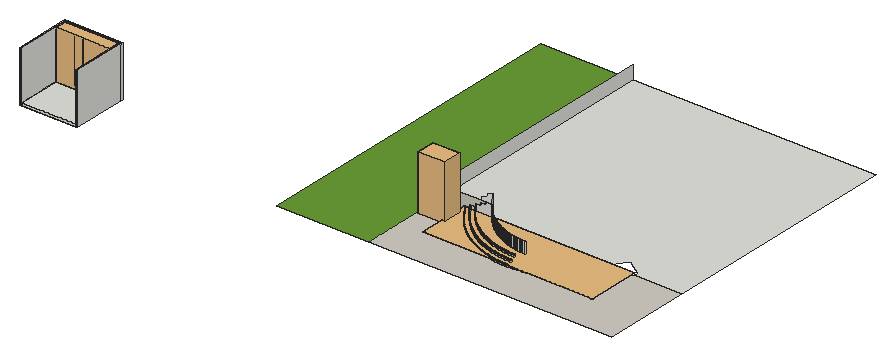
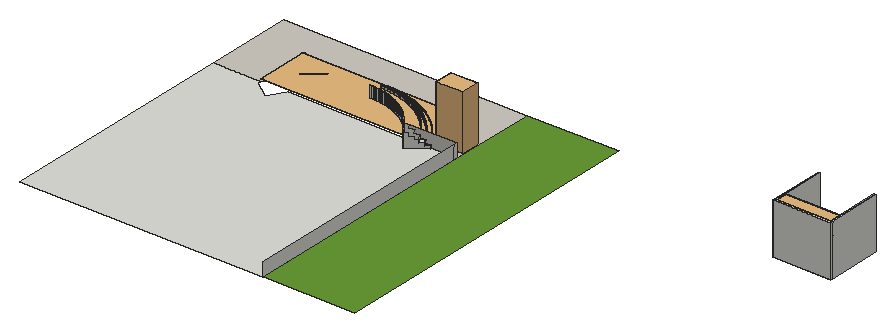
# SketchUp Ruby script. Lengths in inches.
U = 1.inch
M = Sketchup.active_model
def pt(a) = Geom::Point3d.new(a.map { |v| v * U })
def face(e, loops, mat)
  f = e.add_face(loops[0].map { |a| pt(a) })
  loops[1..].each { |l| e.add_face(l.map { |a| pt(a) }).erase! }
  f.material = f.back_material = mat if mat
  f
end
# faces: each face lists its corners as indices into pts; further lists are holes
def faces(e, pts, list, mat = nil) = list.each { |f| face(e, (f[0].is_a?(Array) ? f : [f]).map { |l| l.map { |i| pts[i] } }, mat) }
# xy, xz, yz: faces in a plane at the given z, y or x. An outline is a flat list of corners, or four numbers for a rectangle; further outlines are holes
def ring(l) = l.size == 4 ? [[l[0], l[1]], [l[2], l[1]], [l[2], l[3]], [l[0], l[3]]] : l.each_slice(2).to_a
def flat(e, list, mat, &to3) = list.each { |f| face(e, (f[0].is_a?(Array) ? f : [f]).map { |l| ring(l).map { |u, v| to3.(u, v) } }, mat) }
def xy(e, z, list, mat = nil) = flat(e, list, mat) { |x, y| [x, y, z] }
def xz(e, y, list, mat = nil) = flat(e, list, mat) { |x, z| [x, y, z] }
def yz(e, x, list, mat = nil) = flat(e, list, mat) { |y, z| [x, y, z] }
def lines(e, pts, list) = list.each { |a, b| e.add_line(pt(pts[a]), pt(pts[b])) }
# prism: a flat outline (further loops are holes) pulled along v
def prism(e, loops, v, mat = nil)
  f = face(e, loops, mat); d = Geom::Vector3d.new(v.map { |x| x * U })
  f.pushpull(f.normal.samedirection?(d) ? d.length : -d.length)
end
def box(e, o, s, mat = nil) = prism(e, [[o, [o[0] + s[0], o[1], o[2]], [o[0] + s[0], o[1] + s[1], o[2]], [o[0], o[1] + s[1], o[2]]]], [0, 0, s[2]], mat)
def at(x, y, z, deg = 0) = Geom::Transformation.translation(pt([x, y, z])) * Geom::Transformation.rotation(ORIGIN, Z_AXIS, deg.degrees)
def axes(o, x, y, z) = Geom::Transformation.new([*x, 0, *y, 0, *z, 0, *pt(o).to_a, 1])
def part(name) = M.definitions.add(name)
# library, detail: a bought-in or finely detailed component or shape, given as its bounding box
def library(name, o, s) = part(name).tap { |d| box(d.entities, o, s) }
def detail(e, o, s) = box(e.add_group.entities, o, s)
def put(e, d, t, mat = nil) = e.add_instance(d, t).tap { |i| i.material = mat if mat }
def group(e, t, mat = nil) = e.add_group.tap { |g| g.transformation = t; g.material = mat if mat }.entities
root = M.entities
M.materials.add("Arta-Ceramic-Moonstone-White-24x24-4K").color = [209, 205, 196]
M.materials.add("[Color M09]1").color = [0, 0, 0]
M.materials.add("[Grass Dark Green]").color = [106, 157, 55]
M.materials.add("[Groundcover Gravel 1 inch]").color = [152, 133, 110]
M.materials.add("[Translucent Glass Gray]1").color = [128, 128, 128]
M.materials["[Translucent Glass Gray]1"].alpha = 0.5
c1 = library("Group\#160",[0,-1,0],[120,25,108])
c2 = library("Senza",[-37.85,-41.61,-2.42],[41.39,41.83,53.67])
c3 = library("Mesh Light\#9",[-0.5,-0.5,-0.1],[1,1,0.2])
xy(root,0,[[777.4375,194.875,777.4375,734.875,1318.21,734.875,1318.21,733.875,1318.125,733.875,1318.125,194.875,1212.72,194.875,1216.84,200.64,1177.16,229.03,1152.72,194.875,895.84,194.875,873.77,225.73,834.08,197.34,835.84,194.875],[835.84,194.875,834.08,197.34,873.77,225.73,895.84,194.875]])
xy(root,0,[[[777.4375,0,777.4375,194.875,835.84,194.875,858.18,163.65,860.54,160.49,862.96,157.37,865.43,154.3,867.97,151.27,870.5625,148.3,873.21,145.375,875.92,142.5,878.68,139.68,881.49,136.92,884.36,134.2,887.27,131.55,890.24,128.95,893.26,126.4,896.32,123.92,899.44,121.49,902.59,119.13,905.8,116.82,909.04,114.58,912.33,112.4,915.66,110.29,919.03,108.24,922.44,106.25,925.89,104.33,929.37,102.47,932.89,100.6875,936.44,98.97,940.03,97.32,943.64,95.73,947.29,94.22,950.96,92.78,954.66,91.41,958.38,90.11,962.13,88.88,965.91,87.72,969.7,86.64,973.51,85.63,977.35,84.69,981.2,83.83,985.0625,83.04,988.94,82.32,992.84,81.68,996.74,81.12,1000.66,80.625,1004.58,80.21,1008.51,79.87,1012.45,79.6,1016.39,79.42,1020.34,79.3,1024.28,79.26,1028.23,79.3,1032.17,79.42,1036.11,79.6,1040.05,79.87,1043.98,80.21,1047.9,80.625,1051.82,81.12,1055.72,81.68,1059.62,82.32,1063.5,83.04,1067.36,83.83,1071.21,84.69,1075.05,85.63,1078.86,86.64,1082.66,87.72,1086.43,88.88,1090.18,90.11,1093.9,91.41,1097.6,92.78,1101.28,94.22,1104.92,95.73,1108.54,97.32,1112.12,98.97,1115.67,100.6875,1119.1875,102.47,1122.67,104.33,1126.12,106.25,1129.53,108.24,1132.9,110.29,1136.23,112.4,1139.52,114.58,1142.76,116.82,1145.97,119.13,1149.125,121.49,1152.24,123.92,1155.3,126.4,1158.32,128.95,1161.29,131.55,1164.21,134.2,1167.07,136.92,1169.89,139.68,1172.65,142.5,1175.35,145.375,1178,148.3,1180.59,151.27,1183.13,154.3,1185.6,157.37,1188.02,160.49,1190.38,163.65,1212.72,194.875,1318.125,194.875,1318.125,0],[811.58,149.53,813.26,149.58,814.86,150.07,816.29,150.95,817.44,152.18,818.23,153.66,818.62,155.3,818.5625,156.98,818.08,158.58,817.19,160.01,815.96,161.16,814.48,161.96,812.85,162.34,811.17,162.28,809.56,161.8,808.13,160.91,806.98,159.6875,806.1875,158.2,805.81,156.57,805.86,154.89,806.35,153.28,807.23,151.85,808.46,150.7,809.9375,149.91]]],"Arta-Ceramic-Moonstone-White-24x24-4K")
xy(root,0,[[573.3125,0,777.4375,732.375]],"[Grass Dark Green]")
xy(root,0,[[811.58,149.53,809.9375,149.91,808.46,150.7,807.23,151.85,806.35,153.28,805.86,154.89,805.81,156.57,806.1875,158.2,806.98,159.6875,808.13,160.91,809.56,161.8,811.17,162.28,812.85,162.34,814.48,161.96,815.96,161.16,817.19,160.01,818.08,158.58,818.5625,156.98,818.62,155.3,818.23,153.66,817.44,152.18,816.29,150.95,814.86,150.07,813.26,149.58]],"[Groundcover Gravel 1 inch]")
xy(root,5,[[834.84,194.875,835.5,195.35,835.84,194.875]],"Arta-Ceramic-Moonstone-White-24x24-4K")
xy(root,6,[[835.84,194.875,847.84,194.875,842.02,203.02,834.08,197.34,835.5,195.35]])
xy(root,6,[[834.84,194.875,835.84,194.875,835.5,195.35]],"Arta-Ceramic-Moonstone-White-24x24-4K")
xy(root,11,[[846.84,194.875,847.5,195.35,847.84,194.875]],"Arta-Ceramic-Moonstone-White-24x24-4K")
xy(root,12,[[847.84,194.875,859.84,194.875,849.96,208.69,842.02,203.02,847.5,195.35]])
xy(root,12,[[846.84,194.875,847.84,194.875,847.5,195.35]],"Arta-Ceramic-Moonstone-White-24x24-4K")
xy(root,17,[[858.84,194.875,859.5,195.35,859.84,194.875]],"Arta-Ceramic-Moonstone-White-24x24-4K")
xz(root,194.875,[[835.84,0,895.84,0,895.84,30,882.84,30,882.84,29,883.84,29,883.84,24,870.84,24,870.84,23,871.84,23,871.84,18,858.84,18,858.84,17,859.84,17,859.84,12,846.84,12,846.84,11,847.84,11,847.84,6,834.84,6,834.84,5,835.84,5]])
xz(root,194.875,[[777.4375,0,835.84,0,835.84,5,834.84,5,834.84,6,847.84,6,847.84,11,846.84,11,846.84,12,859.84,12,859.84,17,858.84,17,858.84,18,871.84,18,871.84,23,870.84,23,870.84,24,883.84,24,883.84,29,882.84,29,882.84,30,777.4375,30]],"Arta-Ceramic-Moonstone-White-24x24-4K")
yz(root,777.4375,[[194.875,0,202.125,30],[202.125,0,734.875,30]])
p = [[1016.39,79.42,5],[1016.39,79.42,0],[1020.34,79.3,0],[1020.34,79.3,5],[1024.28,79.26,0],[1024.28,79.26,5],
  [1012.45,79.6,5],[1012.45,79.6,0],[1008.51,79.87,5],[1008.51,79.87,0],[1004.58,80.21,5],[1004.58,80.21,0],
  [1000.66,80.625,5],[1000.66,80.625,0],[996.74,81.12,5],[996.74,81.12,0],[992.84,81.68,5],[992.84,81.68,0],
  [988.94,82.32,5],[988.94,82.32,0],[985.0625,83.04,5],[985.0625,83.04,0],[981.2,83.83,5],[981.2,83.83,0],
  [977.35,84.69,5],[977.35,84.69,0],[973.51,85.63,5],[973.51,85.63,0],[969.7,86.64,5],[969.7,86.64,0],
  [965.91,87.72,5],[965.91,87.72,0],[962.13,88.88,5],[962.13,88.88,0],[958.38,90.11,5],[958.38,90.11,0],
  [954.66,91.41,5],[954.66,91.41,0],[950.96,92.78,5],[950.96,92.78,0],[947.29,94.22,5],[947.29,94.22,0],
  [943.64,95.73,5],[943.64,95.73,0],[940.03,97.32,5],[940.03,97.32,0],[936.44,98.97,5],[936.44,98.97,0],
  [932.89,100.6875,5],[932.89,100.6875,0],[929.37,102.47,5],[929.37,102.47,0],[925.89,104.33,5],[925.89,104.33,0],
  [922.44,106.25,5],[922.44,106.25,0],[919.03,108.24,5],[919.03,108.24,0],[915.66,110.29,5],[915.66,110.29,0],
  [912.33,112.4,5],[912.33,112.4,0],[909.04,114.58,5],[909.04,114.58,0],[905.8,116.82,5],[905.8,116.82,0],
  [902.59,119.13,5],[902.59,119.13,0],[899.44,121.49,5],[899.44,121.49,0],[896.32,123.92,5],[896.32,123.92,0],
  [893.26,126.4,5],[893.26,126.4,0],[890.24,128.95,5],[890.24,128.95,0],[1018.26,128.18,0],[1018.26,128.18,30],
  [1021.27,128.09,30],[1021.27,128.09,0],[1024.28,128.0625,30],[1024.28,128.0625,0],[1015.26,128.32,0],[1015.26,128.32,30],
  [1012.25,128.52,0],[1012.25,128.52,30],[1009.26,128.78,0],[1009.26,128.78,30],[1006.26,129.1,0],[1006.26,129.1,30],
  [887.27,131.55,5],[887.27,131.55,0],[1003.28,129.48,0],[1003.28,129.48,30],[1000.3,129.91,0],[1000.3,129.91,30],
  [997.33,130.4,0],[997.33,130.4,30],[994.37,130.94,0],[994.37,130.94,30],[991.42,131.54,0],[991.42,131.54,30],
  [884.36,134.2,5],[884.36,134.2,0],[988.48,132.2,0],[988.48,132.2,30],[985.56,132.92,0],[985.56,132.92,30],
  [982.65,133.6875,0],[982.65,133.6875,30],[979.76,134.51,0],[979.76,134.51,30],[881.49,136.92,5],[881.49,136.92,0],
  [976.88,135.4,0],[976.88,135.4,30],[974.02,136.33,0],[974.02,136.33,30],[971.18,137.32,0],[971.18,137.32,30],
  [878.68,139.68,5],[878.68,139.68,0],[968.36,138.37,0],[968.36,138.37,30],[965.56,139.47,0],[965.56,139.47,30],
  [962.78,140.625,0],[962.78,140.625,30],[875.92,142.5,5],[875.92,142.5,0],[960.02,141.83,0],[960.02,141.83,30],
  [957.28,143.09,0],[957.28,143.09,30],[873.21,145.375,5],[873.21,145.375,0],[954.58,144.4,0],[954.58,144.4,30],
  [951.89,145.76,0],[951.89,145.76,30],[870.5625,148.3,5],[870.5625,148.3,0],[949.24,147.18,0],[949.24,147.18,30],
  [946.61,148.64,0],[946.61,148.64,30],[867.97,151.27,5],[867.97,151.27,0],[944.01,150.16,0],[944.01,150.16,30],
  [941.4375,151.72,0],[941.4375,151.72,30],[865.43,154.3,5],[865.43,154.3,0],[938.9,153.34,0],[938.9,153.34,30],
  [936.39,155,0],[936.39,155,30],[862.96,157.37,5],[862.96,157.37,0],[933.91,156.71,0],[933.91,156.71,30],
  [931.47,158.47,0],[931.47,158.47,30],[860.54,160.49,5],[860.54,160.49,0],[929.06,160.27,0],[929.06,160.27,30],
  [926.69,162.12,0],[926.69,162.12,30],[858.18,163.65,5],[858.18,163.65,0],[924.35,164.02,0],[924.35,164.02,30],
  [835.84,194.875,5],[835.84,194.875,0],[922.05,165.96,0],[922.05,165.96,30],[919.78,167.94,0],[919.78,167.94,30],
  [917.56,169.97,0],[917.56,169.97,30],[915.37,172.04,0],[915.37,172.04,30],[913.23,174.15,0],[913.23,174.15,30],
  [911.12,176.3,0],[911.12,176.3,30],[909.06,178.49,0],[909.06,178.49,30],[907.04,180.72,0],[907.04,180.72,30],
  [905.06,182.99,0],[905.06,182.99,30],[903.125,185.29,0],[903.125,185.29,30],[901.24,187.64,0],[901.24,187.64,30],
  [899.39,190.01,0],[899.39,190.01,30],[897.59,192.43,0],[897.59,192.43,30],[895.84,194.875,0],[895.84,194.875,30],
  [834.08,197.34,0],[835.5,195.35,5],[835.5,195.35,6],[834.08,197.34,6],[873.77,225.73,0],[873.77,225.73,30],
  [842.02,203.02,6],[842.02,203.02,12],[849.96,208.69,12],[849.96,208.69,18],[857.89,214.375,18],[857.89,214.375,24],
  [865.83,220.05,24],[865.83,220.05,30],[1016.36,78.6,6],[1016.36,78.6,5],[1020.32,78.49,5],[1020.32,78.49,6],
  [1024.28,78.45,5],[1024.28,78.45,6],[1012.4,78.79,6],[1012.4,78.79,5],[1008.45,79.06,6],[1008.45,79.06,5],
  [1004.5,79.4,6],[1004.5,79.4,5],[1000.5625,79.82,6],[1000.5625,79.82,5],[996.63,80.31,6],[996.63,80.31,5],
  [992.71,80.88,6],[992.71,80.88,5],[988.8,81.52,6],[988.8,81.52,5],[984.91,82.24,6],[984.91,82.24,5],
  [981.03,83.03,6],[981.03,83.03,5],[977.16,83.9,6],[977.16,83.9,5],[973.3125,84.84,6],[973.3125,84.84,5],
  [969.48,85.85,6],[969.48,85.85,5],[965.68,86.94,6],[965.68,86.94,5],[961.89,88.1,6],[961.89,88.1,5],
  [958.125,89.34,6],[958.125,89.34,5],[954.38,90.64,6],[954.38,90.64,5],[950.67,92.02,6],[950.67,92.02,5],
  [946.98,93.47,6],[946.98,93.47,5],[943.32,94.99,6],[943.32,94.99,5],[939.69,96.57,6],[939.69,96.57,5],
  [936.09,98.23,6],[936.09,98.23,5],[932.53,99.96,6],[932.53,99.96,5],[929,101.75,6],[929,101.75,5],
  [925.5,103.61,6],[925.5,103.61,5],[922.04,105.54,6],[922.04,105.54,5],[918.62,107.54,6],[918.62,107.54,5],
  [915.23,109.6,6],[915.23,109.6,5],[911.89,111.72,6],[911.89,111.72,5],[908.59,113.91,6],[908.59,113.91,5],
  [905.33,116.16,6],[905.33,116.16,5],[902.11,118.47,6],[902.11,118.47,5],[898.94,120.85,6],[898.94,120.85,5],
  [895.82,123.28,6],[895.82,123.28,5],[892.74,125.78,6],[892.74,125.78,5],[889.71,128.33,6],[889.71,128.33,5],
  [886.73,130.94,6],[886.73,130.94,5],[883.8,133.61,6],[883.8,133.61,5],[880.92,136.33,6],[880.92,136.33,5],
  [878.1,139.11,6],[878.1,139.11,5],[875.33,141.94,6],[875.33,141.94,5],[872.61,144.82,6],[872.61,144.82,5],
  [869.95,147.76,6],[869.95,147.76,5],[867.35,150.75,6],[867.35,150.75,5],[864.81,153.78,6],[864.81,153.78,5],
  [862.32,156.87,6],[862.32,156.87,5],[859.89,160,6],[859.89,160,5],[857.53,163.17,6],[857.53,163.17,5],
  [834.84,194.875,6],[834.84,194.875,5],[1020.52,89.06,11],[1020.52,89.06,6],[1024.28,89.02,6],[1024.28,89.02,11],
  [1016.77,89.17,11],[1016.77,89.17,6],[1013.01,89.35,11],[1013.01,89.35,6],[1009.26,89.6,11],[1009.26,89.6,6],
  [1005.52,89.92,11],[1005.52,89.92,6],[1001.78,90.32,11],[1001.78,90.32,6],[998.05,90.79,11],[998.05,90.79,6],
  [994.33,91.33,11],[994.33,91.33,6],[990.62,91.9375,11],[990.62,91.9375,6],[986.92,92.62,11],[986.92,92.62,6],
  [983.24,93.37,11],[983.24,93.37,6],[979.57,94.19,11],[979.57,94.19,6],[975.92,95.09,11],[975.92,95.09,6],
  [972.29,96.05,11],[972.29,96.05,6],[968.68,97.08,11],[968.68,97.08,6],[965.08,98.18,11],[965.08,98.18,6],
  [961.51,99.35,11],[961.51,99.35,6],[957.96,100.59,11],[957.96,100.59,6],[954.4375,101.9,11],[954.4375,101.9,6],
  [950.9375,103.27,11],[950.9375,103.27,6],[947.47,104.71,11],[947.47,104.71,6],[944.02,106.22,11],[944.02,106.22,6],
  [940.61,107.79,11],[940.61,107.79,6],[937.23,109.43,11],[937.23,109.43,6],[933.875,111.13,11],[933.875,111.13,6],
  [930.56,112.9,11],[930.56,112.9,6],[927.28,114.73,11],[927.28,114.73,6],[924.03,116.62,11],[924.03,116.62,6],
  [920.82,118.57,11],[920.82,118.57,6],[917.65,120.59,11],[917.65,120.59,6],[914.51,122.67,11],[914.51,122.67,6],
  [911.42,124.8,11],[911.42,124.8,6],[908.37,127,11],[908.37,127,6],[905.36,129.25,11],[905.36,129.25,6],
  [902.4,131.56,11],[902.4,131.56,6],[899.48,133.93,11],[899.48,133.93,6],[896.6,136.35,11],[896.6,136.35,6],
  [893.77,138.83,11],[893.77,138.83,6],[891,141.36,11],[891,141.36,6],[888.27,143.94,11],[888.27,143.94,6],
  [885.59,146.58,11],[885.59,146.58,6],[882.96,149.26,11],[882.96,149.26,6],[880.38,152,11],[880.38,152,6],
  [877.86,154.78,11],[877.86,154.78,6],[875.39,157.62,11],[875.39,157.62,6],[872.97,160.5,11],[872.97,160.5,6],
  [870.61,163.42,11],[870.61,163.42,6],[868.31,166.39,11],[868.31,166.39,6],[866.06,169.41,11],[866.06,169.41,6],
  [847.84,194.875,11],[847.84,194.875,6],[847.5,195.35,11],[847.5,195.35,12],[1016.73,88.36,12],[1016.73,88.36,11],
  [1020.51,88.25,11],[1020.51,88.25,12],[1024.28,88.21,11],[1024.28,88.21,12],[1012.96,88.54,12],[1012.96,88.54,11],
  [1009.2,88.79,12],[1009.2,88.79,11],[1005.4375,89.11,12],[1005.4375,89.11,11],[1001.69,89.51,12],[1001.69,89.51,11],
  [997.94,89.98,12],[997.94,89.98,11],[994.21,90.52,12],[994.21,90.52,11],[990.48,91.14,12],[990.48,91.14,11],
  [986.77,91.82,12],[986.77,91.82,11],[983.07,92.58,12],[983.07,92.58,11],[979.39,93.4,12],[979.39,93.4,11],
  [975.72,94.3,12],[975.72,94.3,11],[972.07,95.26,12],[972.07,95.26,11],[968.45,96.3,12],[968.45,96.3,11],
  [964.84,97.41,12],[964.84,97.41,11],[961.25,98.58,12],[961.25,98.58,11],[957.6875,99.83,12],[957.6875,99.83,11],
  [954.15,101.14,12],[954.15,101.14,11],[950.63,102.52,12],[950.63,102.52,11],[947.15,103.96,12],[947.15,103.96,11],
  [943.69,105.48,12],[943.69,105.48,11],[940.26,107.06,12],[940.26,107.06,11],[936.87,108.7,12],[936.87,108.7,11],
  [933.5,110.41,12],[933.5,110.41,11],[930.17,112.18,12],[930.17,112.18,11],[926.875,114.02,12],[926.875,114.02,11],
  [923.61,115.92,12],[923.61,115.92,11],[920.39,117.88,12],[920.39,117.88,11],[917.2,119.91,12],[917.2,119.91,11],
  [914.06,121.99,12],[914.06,121.99,11],[910.95,124.14,12],[910.95,124.14,11],[907.89,126.34,12],[907.89,126.34,11],
  [904.87,128.6,12],[904.87,128.6,11],[901.89,130.92,12],[901.89,130.92,11],[898.96,133.3,12],[898.96,133.3,11],
  [896.07,135.73,12],[896.07,135.73,11],[893.23,138.22,12],[893.23,138.22,11],[890.44,140.76,12],[890.44,140.76,11],
  [887.7,143.35,12],[887.7,143.35,11],[885.01,146,12],[885.01,146,11],[882.37,148.7,12],[882.37,148.7,11],
  [879.78,151.45,12],[879.78,151.45,11],[877.25,154.24,12],[877.25,154.24,11],[874.77,157.09,12],[874.77,157.09,11],
  [872.34,159.98,12],[872.34,159.98,11],[869.97,162.92,12],[869.97,162.92,11],[867.66,165.9,12],[867.66,165.9,11],
  [865.41,168.93,12],[865.41,168.93,11],[846.84,194.875,12],[846.84,194.875,11],[1017.14,98.92,17],[1017.14,98.92,12],
  [1020.71,98.82,12],[1020.71,98.82,17],[1024.28,98.78,12],[1024.28,98.78,17],[1013.57,99.09,17],[1013.57,99.09,12],
  [1010.01,99.33,17],[1010.01,99.33,12],[1006.45,99.64,17],[1006.45,99.64,12],[1002.9,100.02,17],[1002.9,100.02,12],
  [999.36,100.46,17],[999.36,100.46,12],[995.82,100.97,17],[995.82,100.97,12],[992.3,101.55,17],[992.3,101.55,12],
  [988.79,102.2,17],[988.79,102.2,12],[985.29,102.91,17],[985.29,102.91,12],[981.8,103.7,17],[981.8,103.7,12],
  [978.33,104.54,17],[978.33,104.54,12],[974.88,105.46,17],[974.88,105.46,12],[971.45,106.4375,17],[971.45,106.4375,12],
  [968.03,107.49,17],[968.03,107.49,12],[964.64,108.6,17],[964.64,108.6,12],[961.27,109.77,17],[961.27,109.77,12],
  [957.92,111.02,17],[957.92,111.02,12],[954.59,112.32,17],[954.59,112.32,12],[951.29,113.69,17],[951.29,113.69,12],
  [948.02,115.12,17],[948.02,115.12,12],[944.78,116.62,17],[944.78,116.62,12],[941.56,118.17,17],[941.56,118.17,12],
  [938.38,119.79,17],[938.38,119.79,12],[935.23,121.47,17],[935.23,121.47,12],[932.11,123.21,17],[932.11,123.21,12],
  [929.02,125,17],[929.02,125,12],[925.97,126.86,17],[925.97,126.86,12],[922.96,128.78,17],[922.96,128.78,12],
  [919.98,130.75,17],[919.98,130.75,12],[917.04,132.78,17],[917.04,132.78,12],[914.14,134.86,17],[914.14,134.86,12],
  [911.28,137.01,17],[911.28,137.01,12],[908.47,139.2,17],[908.47,139.2,12],[905.69,141.45,17],[905.69,141.45,12],
  [902.96,143.75,17],[902.96,143.75,12],[900.28,146.1,17],[900.28,146.1,12],[897.64,148.51,17],[897.64,148.51,12],
  [895.04,150.96,17],[895.04,150.96,12],[892.5,153.47,17],[892.5,153.47,12],[890,156.02,17],[890,156.02,12],
  [887.55,158.62,17],[887.55,158.62,12],[885.15,161.27,17],[885.15,161.27,12],[882.81,163.96,17],[882.81,163.96,12],
  [880.51,166.7,17],[880.51,166.7,12],[878.27,169.48,17],[878.27,169.48,12],[876.08,172.3,17],[876.08,172.3,12],
  [873.95,175.16,17],[873.95,175.16,12],[859.84,194.875,17],[859.84,194.875,12],[859.5,195.35,17],[859.5,195.35,18],
  [1017.11,98.11,18],[1017.11,98.11,17],[1020.69,98,17],[1020.69,98,18],[1024.28,97.97,17],[1024.28,97.97,18],
  [1013.53,98.28,18],[1013.53,98.28,17],[1009.95,98.52,18],[1009.95,98.52,17],[1006.375,98.83,18],[1006.375,98.83,17],
  [1002.81,99.21,18],[1002.81,99.21,17],[999.25,99.65,18],[999.25,99.65,17],[995.7,100.17,18],[995.7,100.17,17],
  [992.16,100.75,18],[992.16,100.75,17],[988.63,101.4,18],[988.63,101.4,17],[985.12,102.12,18],[985.12,102.12,17],
  [981.62,102.9,18],[981.62,102.9,17],[978.13,103.76,18],[978.13,103.76,17],[974.66,104.67,18],[974.66,104.67,17],
  [971.22,105.66,18],[971.22,105.66,17],[967.79,106.71,18],[967.79,106.71,17],[964.38,107.83,18],[964.38,107.83,17],
  [960.99,109.01,18],[960.99,109.01,17],[957.63,110.26,18],[957.63,110.26,17],[954.29,111.57,18],[954.29,111.57,17],
  [950.98,112.94,18],[950.98,112.94,17],[947.69,114.38,18],[947.69,114.38,17],[944.43,115.88,18],[944.43,115.88,17],
  [941.2,117.44,18],[941.2,117.44,17],[938.01,119.07,18],[938.01,119.07,17],[934.84,120.75,18],[934.84,120.75,17],
  [931.71,122.5,18],[931.71,122.5,17],[928.61,124.31,18],[928.61,124.31,17],[925.54,126.17,18],[925.54,126.17,17],
  [922.52,128.09,18],[922.52,128.09,17],[919.53,130.08,18],[919.53,130.08,17],[916.57,132.11,18],[916.57,132.11,17],
  [913.66,134.21,18],[913.66,134.21,17],[910.79,136.36,18],[910.79,136.36,17],[907.96,138.5625,18],[907.96,138.5625,17],
  [905.18,140.82,18],[905.18,140.82,17],[902.43,143.13,18],[902.43,143.13,17],[899.73,145.5,18],[899.73,145.5,17],
  [897.08,147.91,18],[897.08,147.91,17],[894.48,150.38,18],[894.48,150.38,17],[891.92,152.89,18],[891.92,152.89,17],
  [889.41,155.46,18],[889.41,155.46,17],[886.95,158.07,18],[886.95,158.07,17],[884.54,160.73,18],[884.54,160.73,17],
  [882.1875,163.43,18],[882.1875,163.43,17],[879.88,166.18,18],[879.88,166.18,17],[877.63,168.97,18],[877.63,168.97,17],
  [875.43,171.81,18],[875.43,171.81,17],[873.29,174.68,18],[873.29,174.68,17],[858.84,194.875,18],[858.84,194.875,17]]
faces(root,p,[[0,1,2,3],[3,2,4,5],[6,7,1,0],[8,9,7,6],[10,11,9,8],[12,13,11,10],[14,15,13,12],[16,17,15,14],
  [18,19,17,16],[20,21,19,18],[22,23,21,20],[24,25,23,22],[26,27,25,24],[28,29,27,26],[30,31,29,28],[32,33,31,30],
  [34,35,33,32],[36,37,35,34],[38,39,37,36],[40,41,39,38],[42,43,41,40],[44,45,43,42],[46,47,45,44],[48,49,47,46],
  [50,51,49,48],[52,53,51,50],[54,55,53,52],[56,57,55,54],[58,59,57,56],[60,61,59,58],[62,63,61,60],[64,65,63,62],
  [66,67,65,64],[68,69,67,66],[70,71,69,68],[72,73,71,70],[74,75,73,72],[90,91,75,74],[102,103,91,90],[112,113,103,102],
  [120,121,113,112],[128,129,121,120],[134,135,129,128],[140,141,135,134],[146,147,141,140],[152,153,147,146],[158,159,153,152],[164,165,159,158],
  [170,171,165,164],[174,175,171,170],[218,219,220,221],[221,220,222,223],[224,225,219,218],[226,227,225,224],[228,229,227,226],[230,231,229,228],
  [232,233,231,230],[234,235,233,232],[236,237,235,234],[238,239,237,236],[240,241,239,238],[242,243,241,240],[244,245,243,242],[246,247,245,244],
  [248,249,247,246],[250,251,249,248],[252,253,251,250],[254,255,253,252],[256,257,255,254],[258,259,257,256],[260,261,259,258],[262,263,261,260],
  [264,265,263,262],[266,267,265,264],[268,269,267,266],[270,271,269,268],[272,273,271,270],[274,275,273,272],[276,277,275,274],[278,279,277,276],
  [280,281,279,278],[282,283,281,280],[284,285,283,282],[286,287,285,284],[288,289,287,286],[290,291,289,288],[292,293,291,290],[294,295,293,292],
  [296,297,295,294],[298,299,297,296],[300,301,299,298],[302,303,301,300],[304,305,303,302],[306,307,305,304],[308,309,307,306],[310,311,309,308],
  [312,313,311,310],[314,315,313,312],[316,317,315,314],[316,318,319,317],[205,319,318,206],[320,321,322,323],[324,325,321,320],[326,327,325,324],
  [328,329,327,326],[330,331,329,328],[332,333,331,330],[334,335,333,332],[336,337,335,334],[338,339,337,336],[340,341,339,338],[342,343,341,340],
  [344,345,343,342],[346,347,345,344],[348,349,347,346],[350,351,349,348],[352,353,351,350],[354,355,353,352],[356,357,355,354],[358,359,357,356],
  [360,361,359,358],[362,363,361,360],[364,365,363,362],[366,367,365,364],[368,369,367,366],[370,371,369,368],[372,373,371,370],[374,375,373,372],
  [376,377,375,374],[378,379,377,376],[380,381,379,378],[382,383,381,380],[384,385,383,382],[386,387,385,384],[388,389,387,386],[390,391,389,388],
  [392,393,391,390],[394,395,393,392],[396,397,395,394],[398,399,397,396],[400,401,399,398],[402,403,401,400],[404,405,403,402],[406,407,405,404],
  [408,409,407,406],[410,411,409,408],[412,413,411,410],[414,415,413,412],[416,417,415,414],[418,419,417,416],[420,421,419,418],[424,425,426,427],
  [427,426,428,429],[430,431,425,424],[432,433,431,430],[434,435,433,432],[436,437,435,434],[438,439,437,436],[440,441,439,438],[442,443,441,440],
  [444,445,443,442],[446,447,445,444],[448,449,447,446],[450,451,449,448],[452,453,451,450],[454,455,453,452],[456,457,455,454],[458,459,457,456],
  [460,461,459,458],[462,463,461,460],[464,465,463,462],[466,467,465,464],[468,469,467,466],[470,471,469,468],[472,473,471,470],[474,475,473,472],
  [476,477,475,474],[478,479,477,476],[480,481,479,478],[482,483,481,480],[484,485,483,482],[486,487,485,484],[488,489,487,486],[490,491,489,488],
  [492,493,491,490],[494,495,493,492],[496,497,495,494],[498,499,497,496],[500,501,499,498],[502,503,501,500],[504,505,503,502],[506,507,505,504],
  [508,509,507,506],[510,511,509,508],[512,513,511,510],[514,515,513,512],[516,517,515,514],[518,519,517,516],[520,521,519,518],[522,523,521,520],
  [522,524,525,523],[422,525,524,423],[526,527,528,529],[529,528,530,531],[532,533,527,526],[534,535,533,532],[536,537,535,534],[538,539,537,536],
  [540,541,539,538],[542,543,541,540],[544,545,543,542],[546,547,545,544],[548,549,547,546],[550,551,549,548],[552,553,551,550],[554,555,553,552],
  [556,557,555,554],[558,559,557,556],[560,561,559,558],[562,563,561,560],[564,565,563,562],[566,567,565,564],[568,569,567,566],[570,571,569,568],
  [572,573,571,570],[574,575,573,572],[576,577,575,574],[578,579,577,576],[580,581,579,578],[582,583,581,580],[584,585,583,582],[586,587,585,584],
  [588,589,587,586],[590,591,589,588],[592,593,591,590],[594,595,593,592],[596,597,595,594],[598,599,597,596],[600,601,599,598],[602,603,601,600],
  [604,605,603,602],[606,607,605,604],[608,609,607,606],[610,611,609,608],[612,613,611,610],[614,615,613,612],[616,617,615,614],[618,619,617,616],
  [620,621,619,618],[622,623,621,620],[624,625,623,622],[626,627,625,624],[630,631,632,633],[633,632,634,635],[636,637,631,630],[638,639,637,636],
  [640,641,639,638],[642,643,641,640],[644,645,643,642],[646,647,645,644],[648,649,647,646],[650,651,649,648],[652,653,651,650],[654,655,653,652],
  [656,657,655,654],[658,659,657,656],[660,661,659,658],[662,663,661,660],[664,665,663,662],[666,667,665,664],[668,669,667,666],[670,671,669,668],
  [672,673,671,670],[674,675,673,672],[676,677,675,674],[678,679,677,676],[680,681,679,678],[682,683,681,680],[684,685,683,682],[686,687,685,684],
  [688,689,687,686],[690,691,689,688],[692,693,691,690],[694,695,693,692],[696,697,695,694],[698,699,697,696],[700,701,699,698],[702,703,701,700],
  [704,705,703,702],[706,707,705,704],[708,709,707,706],[710,711,709,708],[712,713,711,710],[714,715,713,712],[716,717,715,714],[718,719,717,716],
  [720,721,719,718],[722,723,721,720],[724,725,723,722],[726,727,725,724],[728,729,727,726],[728,730,731,729],[628,731,730,629]],"Arta-Ceramic-Moonstone-White-24x24-4K")
faces(root,p,[[76,77,78,79],[79,78,80,81],[82,83,77,76],[84,85,83,82],[86,87,85,84],[88,89,87,86],[92,93,89,88],[94,95,93,92],
  [96,97,95,94],[98,99,97,96],[100,101,99,98],[104,105,101,100],[106,107,105,104],[108,109,107,106],[110,111,109,108],[114,115,111,110],
  [116,117,115,114],[118,119,117,116],[122,123,119,118],[124,125,123,122],[126,127,125,124],[130,131,127,126],[132,133,131,130],[136,137,133,132],
  [138,139,137,136],[142,143,139,138],[144,145,143,142],[148,149,145,144],[150,151,149,148],[154,155,151,150],[156,157,155,154],[160,161,157,156],
  [162,163,161,160],[166,167,163,162],[168,169,167,166],[172,173,169,168],[176,177,173,172],[178,179,177,176],[180,181,179,178],[182,183,181,180],
  [184,185,183,182],[186,187,185,184],[188,189,187,186],[190,191,189,188],[192,193,191,190],[194,195,193,192],[196,197,195,194],[198,199,197,196],
  [200,201,199,198],[202,203,201,200],[204,175,174,205,206,207],[203,202,208,209],[207,210,211,212,213,214,215,216,217,209,208,204],[210,421,420,422,423,211],[212,627,626,628,629,213]])
g1 = group(root,at(4.5,0,0))
xy(g1,0,[[-4.5,0,0,120],[0,0,120,120],[120,0,124.5,120],[-4.5,120,124.5,124.5]])
xy(g1,6,[[0,0,120,120]])
xy(g1,114,[[-4.5,0,0,120],[120,0,124.5,120],[-4.5,120,124.5,124.5]])
xz(g1,0,[[-4.5,0,0,114],[0,0,120,6],[120,0,124.5,114]])
xz(g1,120,[[-4.5,0,0,6],[0,0,120,6],[120,0,124.5,6],[-4.5,6,0,114],[0,6,120,114],
  [120,6,124.5,114]])
xz(g1,124.5,[[-4.5,0,124.5,114]])
yz(g1,-4.5,[[0,0,120,114],[120,0,124.5,114]])
yz(g1,0,[[0,0,120,6],[0,6,120,114]])
yz(g1,120,[[0,0,120,6],[0,6,120,114]])
yz(g1,124.5,[[0,0,120,114],[120,0,124.5,114]])
put(root,c1,at(4.5,96,6))
g2 = group(root,at(45.99,96.125,10.71),"[Translucent Glass Gray]1")
xy(g2,0,[[17.86,-0.125,17.86,0,0,0,0,0.24,37.13,0.24,37.13,0,19.39,0,19.39,-0.125,18.68,-0.125,18.68,0,18.57,0,18.57,-0.125]])
xy(g2,101.01,[[17.86,-0.125,18.57,-0.125,18.57,0,18.68,0,18.68,-0.125,19.39,-0.125,19.39,0,37.13,0,37.13,0.24,0,0.24,0,0,17.86,0]])
xz(g2,-0.125,[[17.86,0,18.57,101.01],[18.68,0,19.39,101.01]],"[Color M09]1")
xz(g2,0,[[0,0,17.86,101.01],[19.39,0,37.13,101.01]])
yz(g2,0,[[0,0,0.24,101.01]])
yz(g2,17.86,[[-0.125,0,0,101.01]],"[Color M09]1")
yz(g2,18.57,[[-0.125,0,0,101.01]],"[Color M09]1")
yz(g2,18.68,[[-0.125,0,0,101.01]],"[Color M09]1")
yz(g2,19.39,[[-0.125,0,0,101.01]],"[Color M09]1")
yz(g2,37.13,[[0,0,0.24,101.01]])
put(root,c2,axes([834.95,174.18,0.33],[1.43619,0,0],[0,1,0],[0,0,2.37484]))
g3 = group(root,at(834.84,78.45,5))
xy(g3,0,[[189.4375,0,185.48,0.04,181.52,0.15,177.56,0.34,173.61,0.61,169.66,0.95,165.72,1.37,161.79,1.86,157.87,2.43,153.96,3.07,150.07,3.79,146.18,4.58,142.32,5.45,138.47,6.39,134.64,7.4,130.83,8.49,127.04,9.65,123.28,10.89,119.54,12.19,115.82,13.57,112.14,15.02,108.48,16.53,104.85,18.12,101.25,19.78,97.6875,21.51,94.15,23.3,90.66,25.16,87.2,27.09,83.77,29.09,80.39,31.15,77.05,33.27,73.74,35.46,70.49,37.71,67.27,40.02,64.1,42.4,60.97,44.83,57.9,47.33,54.87,49.88,51.89,52.49,48.96,55.16,46.08,57.88,43.26,60.66,40.49,63.49,37.77,66.375,35.11,69.31,32.51,72.3,29.96,75.33,27.48,78.41,25.05,81.55,22.68,84.72,0,116.42,1,116.42,23.34,85.2,25.7,82.04,28.11,78.92,30.59,75.85,33.125,72.82,35.72,69.85,38.37,66.93,41.07,64.05,43.83,61.23,46.65,58.47,49.51,55.75,52.43,53.1,55.4,50.5,58.41,47.95,61.48,45.47,64.59,43.04,67.75,40.68,70.95,38.375,74.2,36.13,77.49,33.95,80.82,31.84,84.19,29.78,87.6,27.8,91.05,25.875,94.53,24.02,98.05,22.24,101.6,20.52,105.18,18.86,108.8,17.28,112.44,15.77,116.11,14.33,119.81,12.96,123.54,11.66,127.29,10.43,131.0625,9.27,134.86,8.1875,138.67,7.18,142.5,6.24,146.35,5.375,150.22,4.59,154.1,3.87,157.99,3.23,161.9,2.67,165.8125,2.17,169.74,1.76,173.67,1.42,177.61,1.15,181.55,0.96,185.49,0.85,189.4375,0.8125,193.38,0.85,197.33,0.96,201.27,1.15,205.21,1.42,209.14,1.76,213.0625,2.17,216.98,2.67,220.88,3.23,224.77,3.87,228.65,4.59,232.52,5.375,236.37,6.24,240.2,7.18,244.02,8.1875,247.8125,9.27,251.58,10.43,255.33,11.66,259.06,12.96,262.76,14.33,266.43,15.77,270.08,17.28,273.69,18.86,277.28,20.52,280.83,22.24,284.35,24.02,287.83,25.875,291.28,27.8,294.68,29.78,298.05,31.84,301.39,33.95,304.67,36.13,307.92,38.375,311.125,40.68,314.28,43.04,317.4,45.47,320.46,47.95,323.48,50.5,326.45,53.1,329.36,55.75,332.23,58.47,335.04,61.23,337.8,64.05,340.51,66.93,343.16,69.85,345.75,72.82,348.28,75.85,350.76,78.92,353.18,82.04,355.54,85.2,377.875,116.42,378.54,115.95,356.19,84.72,353.83,81.55,351.4,78.41,348.91,75.33,346.37,72.3,343.76,69.31,341.1,66.375,338.39,63.49,335.62,60.66,332.79,57.88,329.92,55.16,326.99,52.49,324.01,49.88,320.98,47.33,317.9,44.83,314.78,42.4,311.61,40.02,308.39,37.71,305.13,35.46,301.83,33.27,298.48,31.15,295.1,29.09,291.68,27.09,288.22,25.16,284.72,23.3,281.1875,21.51,277.625,19.78,274.03,18.12,270.4,16.53,266.74,15.02,263.05,13.57,259.34,12.19,255.6,10.89,251.83,9.65,248.04,8.49,244.23,7.4,240.4,6.39,236.56,5.45,232.69,4.58,228.81,3.79,224.91,3.07,221.01,2.43,217.08,1.86,213.15,1.37,209.21,0.95,205.27,0.61,201.32,0.34,197.36,0.15,193.4,0.04]],"Arta-Ceramic-Moonstone-White-24x24-4K")
put(g3,c3,axes([189.27,58.21,0],[379.53641,0,0],[0,117.42431,0],[0,0,1]))
